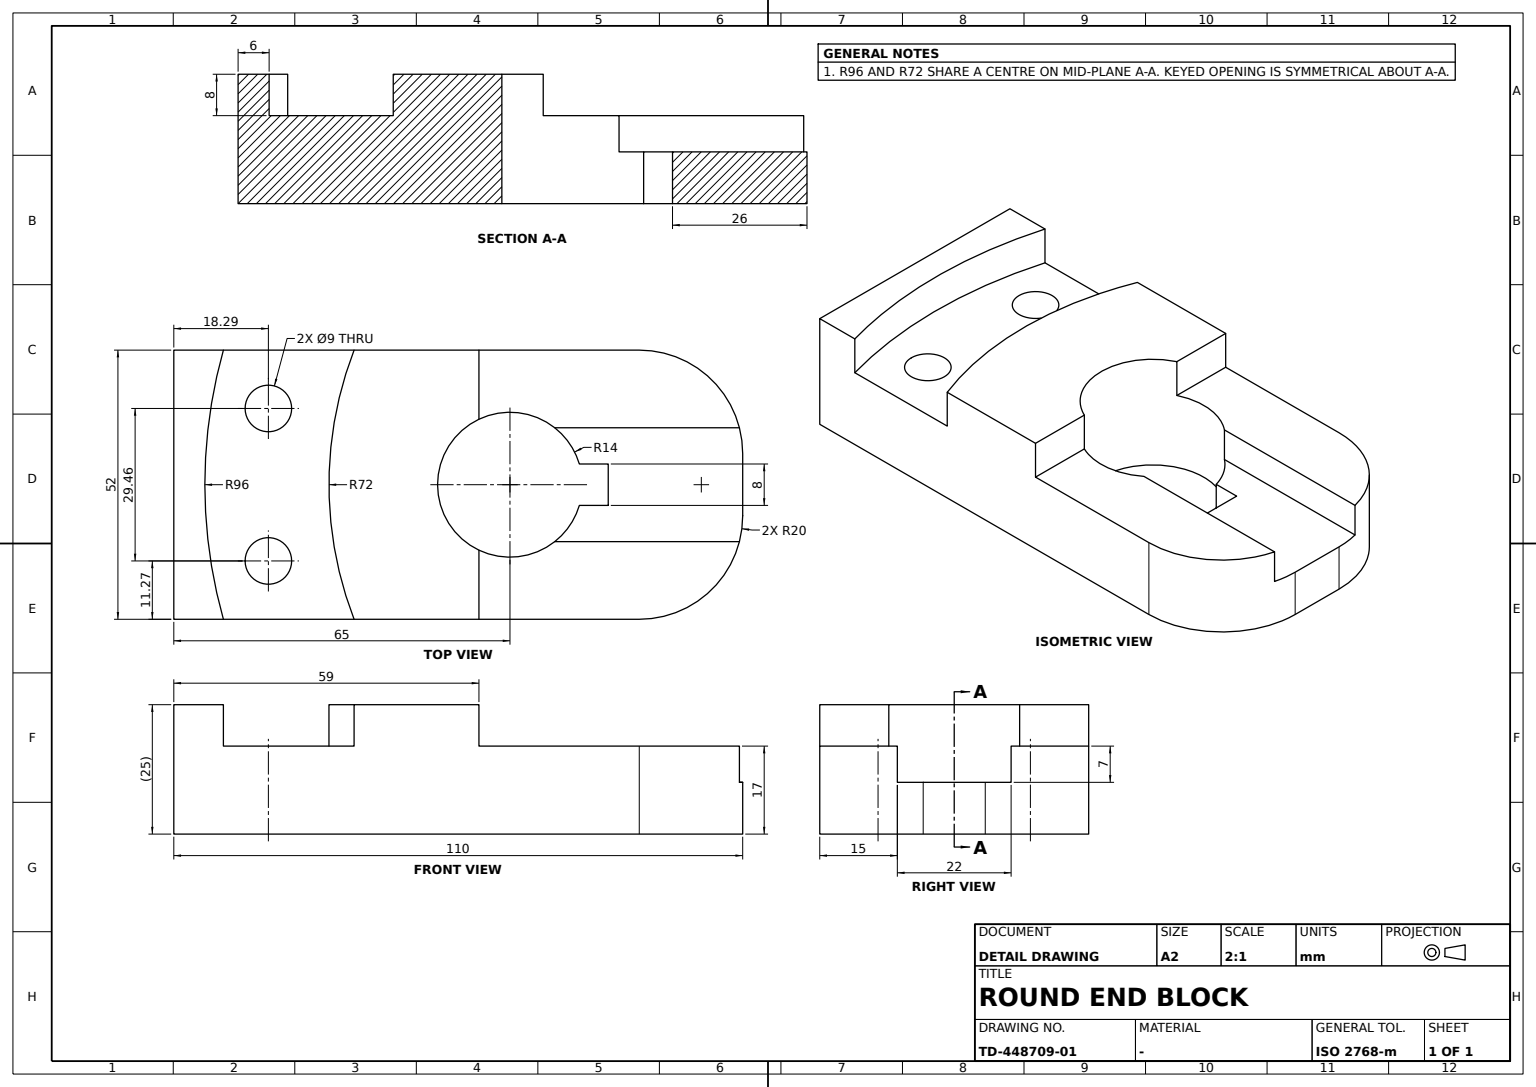
ISO-10303-21;
HEADER;
FILE_DESCRIPTION((''),'2;1');
FILE_NAME('','',(''),(''),'','','');
FILE_SCHEMA(('AUTOMOTIVE_DESIGN'));
ENDSEC;
DATA;
#1=APPLICATION_CONTEXT('');
#2=PRODUCT_CONTEXT('',#1,'mechanical');
#3=PRODUCT('','','',(#2));
#4=PRODUCT_DEFINITION_FORMATION('','',#3);
#5=PRODUCT_DEFINITION_CONTEXT('',#1,'design');
#6=PRODUCT_DEFINITION('','',#4,#5);
#7=PRODUCT_DEFINITION_SHAPE('','',#6);
#8=(LENGTH_UNIT()NAMED_UNIT(*)SI_UNIT(.MILLI.,.METRE.));
#9=(NAMED_UNIT(*)PLANE_ANGLE_UNIT()SI_UNIT($,.RADIAN.));
#10=(NAMED_UNIT(*)SI_UNIT($,.STERADIAN.)SOLID_ANGLE_UNIT());
#11=UNCERTAINTY_MEASURE_WITH_UNIT(LENGTH_MEASURE(0.005),#8,'distance_accuracy_value','');
#12=(GEOMETRIC_REPRESENTATION_CONTEXT(3)GLOBAL_UNCERTAINTY_ASSIGNED_CONTEXT((#11))GLOBAL_UNIT_ASSIGNED_CONTEXT((#8,#9,#10))REPRESENTATION_CONTEXT('',''));
#13=CARTESIAN_POINT('',(22.785849,14.728915,17.));
#14=VERTEX_POINT('',#13);
#15=CARTESIAN_POINT('',(13.785849,14.728915,17.));
#16=VERTEX_POINT('',#15);
#17=CARTESIAN_POINT('',(18.285849,14.728915,17.));
#18=DIRECTION('',(0.,0.,1.));
#19=DIRECTION('',(1.,0.,0.));
#20=AXIS2_PLACEMENT_3D('',#17,#18,#19);
#21=CIRCLE('',#20,4.5);
#22=EDGE_CURVE('',#14,#16,#21,.T.);
#23=ORIENTED_EDGE('',*,*,#22,.T.);
#24=CARTESIAN_POINT('',(13.785849,14.728915,0.));
#25=VERTEX_POINT('',#24);
#26=VECTOR('',#18,1000.);
#27=LINE('',#24,#26);
#28=EDGE_CURVE('',#25,#16,#27,.T.);
#29=ORIENTED_EDGE('',*,*,#28,.F.);
#30=CARTESIAN_POINT('',(22.785849,14.728915,0.));
#31=VERTEX_POINT('',#30);
#32=CARTESIAN_POINT('',(18.285849,14.728915,0.));
#33=AXIS2_PLACEMENT_3D('',#32,#18,#19);
#34=CIRCLE('',#33,4.5);
#35=EDGE_CURVE('',#31,#25,#34,.T.);
#36=ORIENTED_EDGE('',*,*,#35,.F.);
#37=LINE('',#30,#26);
#38=EDGE_CURVE('',#14,#31,#37,.F.);
#39=ORIENTED_EDGE('',*,*,#38,.F.);
#40=EDGE_LOOP('',(#23,#29,#36,#39));
#41=FACE_BOUND('',#40,.T.);
#42=CYLINDRICAL_SURFACE('',#33,4.5);
#43=ADVANCED_FACE('',(#41),#42,.F.);
#44=CARTESIAN_POINT('',(84.,4.,10.));
#45=VERTEX_POINT('',#44);
#46=CARTESIAN_POINT('',(84.,4.,0.));
#47=VERTEX_POINT('',#46);
#48=DIRECTION('',(0.,0.,-1.));
#49=VECTOR('',#48,1000.);
#50=LINE('',#46,#49);
#51=EDGE_CURVE('',#45,#47,#50,.T.);
#52=ORIENTED_EDGE('',*,*,#51,.T.);
#53=CARTESIAN_POINT('',(84.,-4.,0.));
#54=VERTEX_POINT('',#53);
#55=DIRECTION('',(0.,1.,0.));
#56=VECTOR('',#55,1000.);
#57=LINE('',#53,#56);
#58=EDGE_CURVE('',#54,#47,#57,.T.);
#59=ORIENTED_EDGE('',*,*,#58,.F.);
#60=CARTESIAN_POINT('',(84.,-4.,10.));
#61=VERTEX_POINT('',#60);
#62=LINE('',#53,#49);
#63=EDGE_CURVE('',#61,#54,#62,.T.);
#64=ORIENTED_EDGE('',*,*,#63,.F.);
#65=DIRECTION('',(0.,-1.,0.));
#66=VECTOR('',#65,1000.);
#67=LINE('',#60,#66);
#68=EDGE_CURVE('',#45,#61,#67,.T.);
#69=ORIENTED_EDGE('',*,*,#68,.F.);
#70=EDGE_LOOP('',(#52,#59,#64,#69));
#71=FACE_BOUND('',#70,.T.);
#72=AXIS2_PLACEMENT_3D('',#53,#19,#48);
#73=PLANE('',#72);
#74=ADVANCED_FACE('',(#71),#73,.F.);
#75=CARTESIAN_POINT('',(90.,26.,0.));
#76=VERTEX_POINT('',#75);
#77=CARTESIAN_POINT('',(90.,26.,17.));
#78=VERTEX_POINT('',#77);
#79=LINE('',#75,#26);
#80=EDGE_CURVE('',#76,#78,#79,.T.);
#81=ORIENTED_EDGE('',*,*,#80,.T.);
#82=CARTESIAN_POINT('',(109.364917,11.,17.));
#83=VERTEX_POINT('',#82);
#84=CARTESIAN_POINT('',(90.,6.,17.));
#85=AXIS2_PLACEMENT_3D('',#84,#18,#19);
#86=CIRCLE('',#85,20.);
#87=EDGE_CURVE('',#83,#78,#86,.T.);
#88=ORIENTED_EDGE('',*,*,#87,.F.);
#89=CARTESIAN_POINT('',(109.364917,11.,10.));
#90=VERTEX_POINT('',#89);
#91=CARTESIAN_POINT('',(109.364917,11.,0.));
#92=LINE('',#91,#49);
#93=EDGE_CURVE('',#83,#90,#92,.T.);
#94=ORIENTED_EDGE('',*,*,#93,.T.);
#95=CARTESIAN_POINT('',(110.,6.,10.));
#96=VERTEX_POINT('',#95);
#97=CARTESIAN_POINT('',(90.,6.,10.));
#98=AXIS2_PLACEMENT_3D('',#97,#48,#19);
#99=CIRCLE('',#98,20.);
#100=EDGE_CURVE('',#90,#96,#99,.T.);
#101=ORIENTED_EDGE('',*,*,#100,.T.);
#102=CARTESIAN_POINT('',(110.,6.,0.));
#103=VERTEX_POINT('',#102);
#104=LINE('',#102,#26);
#105=EDGE_CURVE('',#103,#96,#104,.T.);
#106=ORIENTED_EDGE('',*,*,#105,.F.);
#107=CARTESIAN_POINT('',(90.,6.,0.));
#108=AXIS2_PLACEMENT_3D('',#107,#18,#19);
#109=CIRCLE('',#108,20.);
#110=EDGE_CURVE('',#103,#76,#109,.T.);
#111=ORIENTED_EDGE('',*,*,#110,.T.);
#112=EDGE_LOOP('',(#81,#88,#94,#101,#106,#111));
#113=FACE_BOUND('',#112,.T.);
#114=CYLINDRICAL_SURFACE('',#108,20.);
#115=ADVANCED_FACE('',(#113),#114,.T.);
#116=CARTESIAN_POINT('',(34.858359,-26.,25.));
#117=VERTEX_POINT('',#116);
#118=CARTESIAN_POINT('',(34.858359,26.,25.));
#119=VERTEX_POINT('',#118);
#120=CARTESIAN_POINT('',(102.,0.,25.));
#121=AXIS2_PLACEMENT_3D('',#120,#48,#19);
#122=CIRCLE('',#121,72.);
#123=EDGE_CURVE('',#117,#119,#122,.T.);
#124=ORIENTED_EDGE('',*,*,#123,.T.);
#125=CARTESIAN_POINT('',(34.858359,26.,17.));
#126=VERTEX_POINT('',#125);
#127=LINE('',#125,#26);
#128=EDGE_CURVE('',#126,#119,#127,.T.);
#129=ORIENTED_EDGE('',*,*,#128,.F.);
#130=CARTESIAN_POINT('',(34.858359,-26.,17.));
#131=VERTEX_POINT('',#130);
#132=CARTESIAN_POINT('',(102.,0.,17.));
#133=AXIS2_PLACEMENT_3D('',#132,#18,#19);
#134=CIRCLE('',#133,72.);
#135=EDGE_CURVE('',#126,#131,#134,.T.);
#136=ORIENTED_EDGE('',*,*,#135,.T.);
#137=LINE('',#130,#26);
#138=EDGE_CURVE('',#131,#117,#137,.T.);
#139=ORIENTED_EDGE('',*,*,#138,.T.);
#140=EDGE_LOOP('',(#124,#129,#136,#139));
#141=FACE_BOUND('',#140,.T.);
#142=CYLINDRICAL_SURFACE('',#133,72.);
#143=ADVANCED_FACE('',(#141),#142,.T.);
#144=CARTESIAN_POINT('',(59.,12.649111,17.));
#145=VERTEX_POINT('',#144);
#146=CARTESIAN_POINT('',(59.,26.,17.));
#147=VERTEX_POINT('',#146);
#148=LINE('',#146,#56);
#149=EDGE_CURVE('',#145,#147,#148,.T.);
#150=ORIENTED_EDGE('',*,*,#149,.T.);
#151=CARTESIAN_POINT('',(59.,26.,25.));
#152=VERTEX_POINT('',#151);
#153=LINE('',#146,#26);
#154=EDGE_CURVE('',#147,#152,#153,.T.);
#155=ORIENTED_EDGE('',*,*,#154,.T.);
#156=CARTESIAN_POINT('',(59.,12.649111,25.));
#157=VERTEX_POINT('',#156);
#158=LINE('',#151,#66);
#159=EDGE_CURVE('',#152,#157,#158,.T.);
#160=ORIENTED_EDGE('',*,*,#159,.T.);
#161=CARTESIAN_POINT('',(59.,12.649111,0.));
#162=LINE('',#161,#26);
#163=EDGE_CURVE('',#145,#157,#162,.T.);
#164=ORIENTED_EDGE('',*,*,#163,.F.);
#165=EDGE_LOOP('',(#150,#155,#160,#164));
#166=FACE_BOUND('',#165,.T.);
#167=DIRECTION('',(-1.,0.,0.));
#168=AXIS2_PLACEMENT_3D('',#146,#167,#18);
#169=PLANE('',#168);
#170=ADVANCED_FACE('',(#166),#169,.F.);
#171=CARTESIAN_POINT('',(73.660254,11.,17.));
#172=VERTEX_POINT('',#171);
#173=CARTESIAN_POINT('',(110.,11.,17.));
#174=VECTOR('',#167,1000.);
#175=LINE('',#173,#174);
#176=EDGE_CURVE('',#83,#172,#175,.T.);
#177=ORIENTED_EDGE('',*,*,#176,.T.);
#178=CARTESIAN_POINT('',(73.660254,11.,10.));
#179=VERTEX_POINT('',#178);
#180=LINE('',#171,#49);
#181=EDGE_CURVE('',#172,#179,#180,.T.);
#182=ORIENTED_EDGE('',*,*,#181,.T.);
#183=CARTESIAN_POINT('',(110.,11.,10.));
#184=VECTOR('',#19,1000.);
#185=LINE('',#183,#184);
#186=EDGE_CURVE('',#179,#90,#185,.T.);
#187=ORIENTED_EDGE('',*,*,#186,.T.);
#188=ORIENTED_EDGE('',*,*,#93,.F.);
#189=EDGE_LOOP('',(#177,#182,#187,#188));
#190=FACE_BOUND('',#189,.T.);
#191=AXIS2_PLACEMENT_3D('',#173,#65,#19);
#192=PLANE('',#191);
#193=ADVANCED_FACE('',(#190),#192,.T.);
#194=CARTESIAN_POINT('',(9.58788,26.,25.));
#195=VERTEX_POINT('',#194);
#196=CARTESIAN_POINT('',(9.58788,-26.,25.));
#197=VERTEX_POINT('',#196);
#198=AXIS2_PLACEMENT_3D('',#120,#18,#19);
#199=CIRCLE('',#198,96.);
#200=EDGE_CURVE('',#195,#197,#199,.T.);
#201=ORIENTED_EDGE('',*,*,#200,.T.);
#202=CARTESIAN_POINT('',(9.58788,-26.,17.));
#203=VERTEX_POINT('',#202);
#204=LINE('',#202,#26);
#205=EDGE_CURVE('',#203,#197,#204,.T.);
#206=ORIENTED_EDGE('',*,*,#205,.F.);
#207=CARTESIAN_POINT('',(9.58788,26.,17.));
#208=VERTEX_POINT('',#207);
#209=AXIS2_PLACEMENT_3D('',#132,#48,#19);
#210=CIRCLE('',#209,96.);
#211=EDGE_CURVE('',#203,#208,#210,.T.);
#212=ORIENTED_EDGE('',*,*,#211,.T.);
#213=LINE('',#207,#26);
#214=EDGE_CURVE('',#208,#195,#213,.T.);
#215=ORIENTED_EDGE('',*,*,#214,.T.);
#216=EDGE_LOOP('',(#201,#206,#212,#215));
#217=FACE_BOUND('',#216,.T.);
#218=CYLINDRICAL_SURFACE('',#133,96.);
#219=ADVANCED_FACE('',(#217),#218,.F.);
#220=ORIENTED_EDGE('',*,*,#123,.F.);
#221=CARTESIAN_POINT('',(59.,-26.,25.));
#222=VERTEX_POINT('',#221);
#223=CARTESIAN_POINT('',(0.,-26.,25.));
#224=LINE('',#223,#184);
#225=EDGE_CURVE('',#117,#222,#224,.T.);
#226=ORIENTED_EDGE('',*,*,#225,.T.);
#227=CARTESIAN_POINT('',(59.,-12.649111,25.));
#228=VERTEX_POINT('',#227);
#229=EDGE_CURVE('',#228,#222,#158,.T.);
#230=ORIENTED_EDGE('',*,*,#229,.F.);
#231=CARTESIAN_POINT('',(65.,0.,25.));
#232=AXIS2_PLACEMENT_3D('',#231,#18,#19);
#233=CIRCLE('',#232,14.);
#234=EDGE_CURVE('',#157,#228,#233,.T.);
#235=ORIENTED_EDGE('',*,*,#234,.F.);
#236=ORIENTED_EDGE('',*,*,#159,.F.);
#237=CARTESIAN_POINT('',(90.,26.,25.));
#238=LINE('',#237,#174);
#239=EDGE_CURVE('',#152,#119,#238,.T.);
#240=ORIENTED_EDGE('',*,*,#239,.T.);
#241=EDGE_LOOP('',(#220,#226,#230,#235,#236,#240));
#242=FACE_BOUND('',#241,.T.);
#243=CARTESIAN_POINT('',(90.,-6.,25.));
#244=AXIS2_PLACEMENT_3D('',#243,#18,#19);
#245=PLANE('',#244);
#246=ADVANCED_FACE('',(#242),#245,.T.);
#247=CARTESIAN_POINT('',(110.,-6.,0.));
#248=VERTEX_POINT('',#247);
#249=CARTESIAN_POINT('',(110.,-6.,10.));
#250=VERTEX_POINT('',#249);
#251=LINE('',#247,#26);
#252=EDGE_CURVE('',#248,#250,#251,.T.);
#253=ORIENTED_EDGE('',*,*,#252,.F.);
#254=LINE('',#247,#56);
#255=EDGE_CURVE('',#248,#103,#254,.T.);
#256=ORIENTED_EDGE('',*,*,#255,.T.);
#257=ORIENTED_EDGE('',*,*,#105,.T.);
#258=CARTESIAN_POINT('',(110.,-11.,10.));
#259=LINE('',#258,#56);
#260=EDGE_CURVE('',#250,#96,#259,.T.);
#261=ORIENTED_EDGE('',*,*,#260,.F.);
#262=EDGE_LOOP('',(#253,#256,#257,#261));
#263=FACE_BOUND('',#262,.T.);
#264=AXIS2_PLACEMENT_3D('',#247,#19,#48);
#265=PLANE('',#264);
#266=ADVANCED_FACE('',(#263),#265,.T.);
#267=CARTESIAN_POINT('',(78.416408,-4.,10.));
#268=VERTEX_POINT('',#267);
#269=LINE('',#267,#174);
#270=EDGE_CURVE('',#61,#268,#269,.T.);
#271=ORIENTED_EDGE('',*,*,#270,.F.);
#272=ORIENTED_EDGE('',*,*,#63,.T.);
#273=CARTESIAN_POINT('',(78.416408,-4.,0.));
#274=VERTEX_POINT('',#273);
#275=LINE('',#273,#184);
#276=EDGE_CURVE('',#274,#54,#275,.T.);
#277=ORIENTED_EDGE('',*,*,#276,.F.);
#278=LINE('',#273,#49);
#279=EDGE_CURVE('',#268,#274,#278,.T.);
#280=ORIENTED_EDGE('',*,*,#279,.F.);
#281=EDGE_LOOP('',(#271,#272,#277,#280));
#282=FACE_BOUND('',#281,.T.);
#283=AXIS2_PLACEMENT_3D('',#273,#65,#48);
#284=PLANE('',#283);
#285=ADVANCED_FACE('',(#282),#284,.F.);
#286=CARTESIAN_POINT('',(90.,-26.,0.));
#287=VERTEX_POINT('',#286);
#288=CARTESIAN_POINT('',(90.,-6.,0.));
#289=AXIS2_PLACEMENT_3D('',#288,#18,#19);
#290=CIRCLE('',#289,20.);
#291=EDGE_CURVE('',#287,#248,#290,.T.);
#292=ORIENTED_EDGE('',*,*,#291,.T.);
#293=ORIENTED_EDGE('',*,*,#252,.T.);
#294=CARTESIAN_POINT('',(109.364917,-11.,10.));
#295=VERTEX_POINT('',#294);
#296=CARTESIAN_POINT('',(90.,-6.,10.));
#297=AXIS2_PLACEMENT_3D('',#296,#48,#19);
#298=CIRCLE('',#297,20.);
#299=EDGE_CURVE('',#250,#295,#298,.T.);
#300=ORIENTED_EDGE('',*,*,#299,.T.);
#301=CARTESIAN_POINT('',(109.364917,-11.,17.));
#302=VERTEX_POINT('',#301);
#303=CARTESIAN_POINT('',(109.364917,-11.,0.));
#304=LINE('',#303,#26);
#305=EDGE_CURVE('',#295,#302,#304,.T.);
#306=ORIENTED_EDGE('',*,*,#305,.T.);
#307=CARTESIAN_POINT('',(90.,-26.,17.));
#308=VERTEX_POINT('',#307);
#309=CARTESIAN_POINT('',(90.,-6.,17.));
#310=AXIS2_PLACEMENT_3D('',#309,#18,#19);
#311=CIRCLE('',#310,20.);
#312=EDGE_CURVE('',#308,#302,#311,.T.);
#313=ORIENTED_EDGE('',*,*,#312,.F.);
#314=LINE('',#286,#26);
#315=EDGE_CURVE('',#287,#308,#314,.T.);
#316=ORIENTED_EDGE('',*,*,#315,.F.);
#317=EDGE_LOOP('',(#292,#293,#300,#306,#313,#316));
#318=FACE_BOUND('',#317,.T.);
#319=CYLINDRICAL_SURFACE('',#289,20.);
#320=ADVANCED_FACE('',(#318),#319,.T.);
#321=ORIENTED_EDGE('',*,*,#270,.T.);
#322=CARTESIAN_POINT('',(73.660254,-11.,10.));
#323=VERTEX_POINT('',#322);
#324=CARTESIAN_POINT('',(65.,0.,10.));
#325=AXIS2_PLACEMENT_3D('',#324,#48,#19);
#326=CIRCLE('',#325,14.);
#327=EDGE_CURVE('',#268,#323,#326,.T.);
#328=ORIENTED_EDGE('',*,*,#327,.T.);
#329=LINE('',#322,#174);
#330=EDGE_CURVE('',#295,#323,#329,.T.);
#331=ORIENTED_EDGE('',*,*,#330,.F.);
#332=ORIENTED_EDGE('',*,*,#299,.F.);
#333=ORIENTED_EDGE('',*,*,#260,.T.);
#334=ORIENTED_EDGE('',*,*,#100,.F.);
#335=ORIENTED_EDGE('',*,*,#186,.F.);
#336=CARTESIAN_POINT('',(78.416408,4.,10.));
#337=VERTEX_POINT('',#336);
#338=EDGE_CURVE('',#179,#337,#326,.T.);
#339=ORIENTED_EDGE('',*,*,#338,.T.);
#340=LINE('',#44,#184);
#341=EDGE_CURVE('',#337,#45,#340,.T.);
#342=ORIENTED_EDGE('',*,*,#341,.T.);
#343=ORIENTED_EDGE('',*,*,#68,.T.);
#344=EDGE_LOOP('',(#321,#328,#331,#332,#333,#334,#335,#339,#342,#343));
#345=FACE_BOUND('',#344,.T.);
#346=CARTESIAN_POINT('',(0.,0.,10.));
#347=AXIS2_PLACEMENT_3D('',#346,#18,#19);
#348=PLANE('',#347);
#349=ADVANCED_FACE('',(#345),#348,.T.);
#350=CARTESIAN_POINT('',(59.,-26.,17.));
#351=VERTEX_POINT('',#350);
#352=LINE('',#350,#26);
#353=EDGE_CURVE('',#351,#222,#352,.T.);
#354=ORIENTED_EDGE('',*,*,#353,.T.);
#355=ORIENTED_EDGE('',*,*,#225,.F.);
#356=ORIENTED_EDGE('',*,*,#138,.F.);
#357=LINE('',#202,#184);
#358=EDGE_CURVE('',#203,#131,#357,.T.);
#359=ORIENTED_EDGE('',*,*,#358,.F.);
#360=ORIENTED_EDGE('',*,*,#205,.T.);
#361=VERTEX_POINT('',#223);
#362=EDGE_CURVE('',#361,#197,#224,.T.);
#363=ORIENTED_EDGE('',*,*,#362,.F.);
#364=CARTESIAN_POINT('',(0.,-26.,0.));
#365=VERTEX_POINT('',#364);
#366=LINE('',#364,#26);
#367=EDGE_CURVE('',#365,#361,#366,.T.);
#368=ORIENTED_EDGE('',*,*,#367,.F.);
#369=LINE('',#364,#184);
#370=EDGE_CURVE('',#365,#287,#369,.T.);
#371=ORIENTED_EDGE('',*,*,#370,.T.);
#372=ORIENTED_EDGE('',*,*,#315,.T.);
#373=LINE('',#350,#184);
#374=EDGE_CURVE('',#351,#308,#373,.T.);
#375=ORIENTED_EDGE('',*,*,#374,.F.);
#376=EDGE_LOOP('',(#354,#355,#356,#359,#360,#363,#368,#371,#372,#375));
#377=FACE_BOUND('',#376,.T.);
#378=AXIS2_PLACEMENT_3D('',#364,#65,#48);
#379=PLANE('',#378);
#380=ADVANCED_FACE('',(#377),#379,.T.);
#381=CARTESIAN_POINT('',(13.785849,-14.728915,17.));
#382=VERTEX_POINT('',#381);
#383=CARTESIAN_POINT('',(22.785849,-14.728915,17.));
#384=VERTEX_POINT('',#383);
#385=CARTESIAN_POINT('',(18.285849,-14.728915,17.));
#386=AXIS2_PLACEMENT_3D('',#385,#18,#19);
#387=CIRCLE('',#386,4.5);
#388=EDGE_CURVE('',#382,#384,#387,.T.);
#389=ORIENTED_EDGE('',*,*,#388,.T.);
#390=CARTESIAN_POINT('',(22.785849,-14.728915,0.));
#391=VERTEX_POINT('',#390);
#392=LINE('',#390,#26);
#393=EDGE_CURVE('',#391,#384,#392,.T.);
#394=ORIENTED_EDGE('',*,*,#393,.F.);
#395=CARTESIAN_POINT('',(13.785849,-14.728915,0.));
#396=VERTEX_POINT('',#395);
#397=CARTESIAN_POINT('',(18.285849,-14.728915,0.));
#398=AXIS2_PLACEMENT_3D('',#397,#18,#19);
#399=CIRCLE('',#398,4.5);
#400=EDGE_CURVE('',#396,#391,#399,.T.);
#401=ORIENTED_EDGE('',*,*,#400,.F.);
#402=LINE('',#395,#26);
#403=EDGE_CURVE('',#382,#396,#402,.F.);
#404=ORIENTED_EDGE('',*,*,#403,.F.);
#405=EDGE_LOOP('',(#389,#394,#401,#404));
#406=FACE_BOUND('',#405,.T.);
#407=CYLINDRICAL_SURFACE('',#398,4.5);
#408=ADVANCED_FACE('',(#406),#407,.F.);
#409=ORIENTED_EDGE('',*,*,#341,.F.);
#410=CARTESIAN_POINT('',(78.416408,4.,0.));
#411=VERTEX_POINT('',#410);
#412=LINE('',#410,#49);
#413=EDGE_CURVE('',#337,#411,#412,.T.);
#414=ORIENTED_EDGE('',*,*,#413,.T.);
#415=LINE('',#46,#174);
#416=EDGE_CURVE('',#47,#411,#415,.T.);
#417=ORIENTED_EDGE('',*,*,#416,.F.);
#418=ORIENTED_EDGE('',*,*,#51,.F.);
#419=EDGE_LOOP('',(#409,#414,#417,#418));
#420=FACE_BOUND('',#419,.T.);
#421=AXIS2_PLACEMENT_3D('',#46,#55,#18);
#422=PLANE('',#421);
#423=ADVANCED_FACE('',(#420),#422,.F.);
#424=CARTESIAN_POINT('',(73.660254,-11.,17.));
#425=VERTEX_POINT('',#424);
#426=LINE('',#424,#49);
#427=EDGE_CURVE('',#425,#323,#426,.T.);
#428=ORIENTED_EDGE('',*,*,#427,.F.);
#429=LINE('',#424,#184);
#430=EDGE_CURVE('',#425,#302,#429,.T.);
#431=ORIENTED_EDGE('',*,*,#430,.T.);
#432=ORIENTED_EDGE('',*,*,#305,.F.);
#433=ORIENTED_EDGE('',*,*,#330,.T.);
#434=EDGE_LOOP('',(#428,#431,#432,#433));
#435=FACE_BOUND('',#434,.T.);
#436=AXIS2_PLACEMENT_3D('',#424,#55,#167);
#437=PLANE('',#436);
#438=ADVANCED_FACE('',(#435),#437,.T.);
#439=CARTESIAN_POINT('',(59.,-12.649111,17.));
#440=VERTEX_POINT('',#439);
#441=CARTESIAN_POINT('',(59.,-12.649111,0.));
#442=LINE('',#441,#49);
#443=EDGE_CURVE('',#228,#440,#442,.T.);
#444=ORIENTED_EDGE('',*,*,#443,.F.);
#445=ORIENTED_EDGE('',*,*,#229,.T.);
#446=ORIENTED_EDGE('',*,*,#353,.F.);
#447=EDGE_CURVE('',#351,#440,#148,.T.);
#448=ORIENTED_EDGE('',*,*,#447,.T.);
#449=EDGE_LOOP('',(#444,#445,#446,#448));
#450=FACE_BOUND('',#449,.T.);
#451=ADVANCED_FACE('',(#450),#169,.F.);
#452=EDGE_CURVE('',#391,#396,#399,.T.);
#453=ORIENTED_EDGE('',*,*,#452,.F.);
#454=ORIENTED_EDGE('',*,*,#393,.T.);
#455=EDGE_CURVE('',#384,#382,#387,.T.);
#456=ORIENTED_EDGE('',*,*,#455,.T.);
#457=ORIENTED_EDGE('',*,*,#403,.T.);
#458=EDGE_LOOP('',(#453,#454,#456,#457));
#459=FACE_BOUND('',#458,.T.);
#460=ADVANCED_FACE('',(#459),#407,.F.);
#461=ORIENTED_EDGE('',*,*,#87,.T.);
#462=LINE('',#77,#174);
#463=EDGE_CURVE('',#78,#147,#462,.T.);
#464=ORIENTED_EDGE('',*,*,#463,.T.);
#465=ORIENTED_EDGE('',*,*,#149,.F.);
#466=CARTESIAN_POINT('',(65.,0.,17.));
#467=AXIS2_PLACEMENT_3D('',#466,#48,#19);
#468=CIRCLE('',#467,14.);
#469=EDGE_CURVE('',#145,#172,#468,.T.);
#470=ORIENTED_EDGE('',*,*,#469,.T.);
#471=ORIENTED_EDGE('',*,*,#176,.F.);
#472=EDGE_LOOP('',(#461,#464,#465,#470,#471));
#473=FACE_BOUND('',#472,.T.);
#474=PLANE('',#310);
#475=ADVANCED_FACE('',(#473),#474,.T.);
#476=CARTESIAN_POINT('',(0.,26.,0.));
#477=VERTEX_POINT('',#476);
#478=CARTESIAN_POINT('',(0.,26.,25.));
#479=VERTEX_POINT('',#478);
#480=LINE('',#476,#26);
#481=EDGE_CURVE('',#477,#479,#480,.T.);
#482=ORIENTED_EDGE('',*,*,#481,.F.);
#483=LINE('',#476,#66);
#484=EDGE_CURVE('',#477,#365,#483,.T.);
#485=ORIENTED_EDGE('',*,*,#484,.T.);
#486=ORIENTED_EDGE('',*,*,#367,.T.);
#487=LINE('',#478,#66);
#488=EDGE_CURVE('',#479,#361,#487,.T.);
#489=ORIENTED_EDGE('',*,*,#488,.F.);
#490=EDGE_LOOP('',(#482,#485,#486,#489));
#491=FACE_BOUND('',#490,.T.);
#492=AXIS2_PLACEMENT_3D('',#476,#167,#18);
#493=PLANE('',#492);
#494=ADVANCED_FACE('',(#491),#493,.T.);
#495=ORIENTED_EDGE('',*,*,#35,.T.);
#496=EDGE_CURVE('',#25,#31,#34,.T.);
#497=ORIENTED_EDGE('',*,*,#496,.T.);
#498=EDGE_LOOP('',(#495,#497));
#499=FACE_BOUND('',#498,.T.);
#500=ORIENTED_EDGE('',*,*,#452,.T.);
#501=ORIENTED_EDGE('',*,*,#400,.T.);
#502=EDGE_LOOP('',(#500,#501));
#503=FACE_BOUND('',#502,.T.);
#504=ORIENTED_EDGE('',*,*,#416,.T.);
#505=CARTESIAN_POINT('',(65.,0.,0.));
#506=AXIS2_PLACEMENT_3D('',#505,#18,#19);
#507=CIRCLE('',#506,14.);
#508=EDGE_CURVE('',#411,#274,#507,.T.);
#509=ORIENTED_EDGE('',*,*,#508,.T.);
#510=ORIENTED_EDGE('',*,*,#276,.T.);
#511=ORIENTED_EDGE('',*,*,#58,.T.);
#512=EDGE_LOOP('',(#504,#509,#510,#511));
#513=FACE_BOUND('',#512,.T.);
#514=ORIENTED_EDGE('',*,*,#484,.F.);
#515=LINE('',#75,#174);
#516=EDGE_CURVE('',#76,#477,#515,.T.);
#517=ORIENTED_EDGE('',*,*,#516,.F.);
#518=ORIENTED_EDGE('',*,*,#110,.F.);
#519=ORIENTED_EDGE('',*,*,#255,.F.);
#520=ORIENTED_EDGE('',*,*,#291,.F.);
#521=ORIENTED_EDGE('',*,*,#370,.F.);
#522=EDGE_LOOP('',(#514,#517,#518,#519,#520,#521));
#523=FACE_BOUND('',#522,.T.);
#524=PLANE('',#289);
#525=ADVANCED_FACE('',(#499,#503,#513,#523),#524,.F.);
#526=ORIENTED_EDGE('',*,*,#488,.T.);
#527=ORIENTED_EDGE('',*,*,#362,.T.);
#528=ORIENTED_EDGE('',*,*,#200,.F.);
#529=EDGE_CURVE('',#195,#479,#238,.T.);
#530=ORIENTED_EDGE('',*,*,#529,.T.);
#531=EDGE_LOOP('',(#526,#527,#528,#530));
#532=FACE_BOUND('',#531,.T.);
#533=ADVANCED_FACE('',(#532),#245,.T.);
#534=ORIENTED_EDGE('',*,*,#447,.F.);
#535=ORIENTED_EDGE('',*,*,#374,.T.);
#536=ORIENTED_EDGE('',*,*,#312,.T.);
#537=ORIENTED_EDGE('',*,*,#430,.F.);
#538=EDGE_CURVE('',#425,#440,#468,.T.);
#539=ORIENTED_EDGE('',*,*,#538,.T.);
#540=EDGE_LOOP('',(#534,#535,#536,#537,#539));
#541=FACE_BOUND('',#540,.T.);
#542=ADVANCED_FACE('',(#541),#474,.T.);
#543=ORIENTED_EDGE('',*,*,#443,.T.);
#544=ORIENTED_EDGE('',*,*,#538,.F.);
#545=ORIENTED_EDGE('',*,*,#427,.T.);
#546=ORIENTED_EDGE('',*,*,#327,.F.);
#547=ORIENTED_EDGE('',*,*,#279,.T.);
#548=ORIENTED_EDGE('',*,*,#508,.F.);
#549=ORIENTED_EDGE('',*,*,#413,.F.);
#550=ORIENTED_EDGE('',*,*,#338,.F.);
#551=ORIENTED_EDGE('',*,*,#181,.F.);
#552=ORIENTED_EDGE('',*,*,#469,.F.);
#553=ORIENTED_EDGE('',*,*,#163,.T.);
#554=ORIENTED_EDGE('',*,*,#234,.T.);
#555=EDGE_LOOP('',(#543,#544,#545,#546,#547,#548,#549,#550,#551,#552,#553,#554));
#556=FACE_BOUND('',#555,.T.);
#557=CYLINDRICAL_SURFACE('',#506,14.);
#558=ADVANCED_FACE('',(#556),#557,.F.);
#559=EDGE_CURVE('',#16,#14,#21,.T.);
#560=ORIENTED_EDGE('',*,*,#559,.T.);
#561=ORIENTED_EDGE('',*,*,#38,.T.);
#562=ORIENTED_EDGE('',*,*,#496,.F.);
#563=ORIENTED_EDGE('',*,*,#28,.T.);
#564=EDGE_LOOP('',(#560,#561,#562,#563));
#565=FACE_BOUND('',#564,.T.);
#566=ADVANCED_FACE('',(#565),#42,.F.);
#567=ORIENTED_EDGE('',*,*,#516,.T.);
#568=ORIENTED_EDGE('',*,*,#481,.T.);
#569=ORIENTED_EDGE('',*,*,#529,.F.);
#570=ORIENTED_EDGE('',*,*,#214,.F.);
#571=LINE('',#125,#174);
#572=EDGE_CURVE('',#126,#208,#571,.T.);
#573=ORIENTED_EDGE('',*,*,#572,.F.);
#574=ORIENTED_EDGE('',*,*,#128,.T.);
#575=ORIENTED_EDGE('',*,*,#239,.F.);
#576=ORIENTED_EDGE('',*,*,#154,.F.);
#577=ORIENTED_EDGE('',*,*,#463,.F.);
#578=ORIENTED_EDGE('',*,*,#80,.F.);
#579=EDGE_LOOP('',(#567,#568,#569,#570,#573,#574,#575,#576,#577,#578));
#580=FACE_BOUND('',#579,.T.);
#581=AXIS2_PLACEMENT_3D('',#75,#55,#18);
#582=PLANE('',#581);
#583=ADVANCED_FACE('',(#580),#582,.T.);
#584=ORIENTED_EDGE('',*,*,#455,.F.);
#585=ORIENTED_EDGE('',*,*,#388,.F.);
#586=EDGE_LOOP('',(#584,#585));
#587=FACE_BOUND('',#586,.T.);
#588=ORIENTED_EDGE('',*,*,#559,.F.);
#589=ORIENTED_EDGE('',*,*,#22,.F.);
#590=EDGE_LOOP('',(#588,#589));
#591=FACE_BOUND('',#590,.T.);
#592=ORIENTED_EDGE('',*,*,#135,.F.);
#593=ORIENTED_EDGE('',*,*,#572,.T.);
#594=ORIENTED_EDGE('',*,*,#211,.F.);
#595=ORIENTED_EDGE('',*,*,#358,.T.);
#596=EDGE_LOOP('',(#592,#593,#594,#595));
#597=FACE_BOUND('',#596,.T.);
#598=PLANE('',#133);
#599=ADVANCED_FACE('',(#587,#591,#597),#598,.T.);
#600=CLOSED_SHELL('',(#43,#74,#115,#143,#170,#193,#219,#246,#266,#285,#320,#349,#380,#408,#423,#438,#451,#460,#475,#494,#525,#533,#542,#558,#566,#583,#599));
#601=MANIFOLD_SOLID_BREP('',#600);
#602=ADVANCED_BREP_SHAPE_REPRESENTATION('',(#601),#12);
#603=SHAPE_DEFINITION_REPRESENTATION(#7,#602);
ENDSEC;
END-ISO-10303-21;
